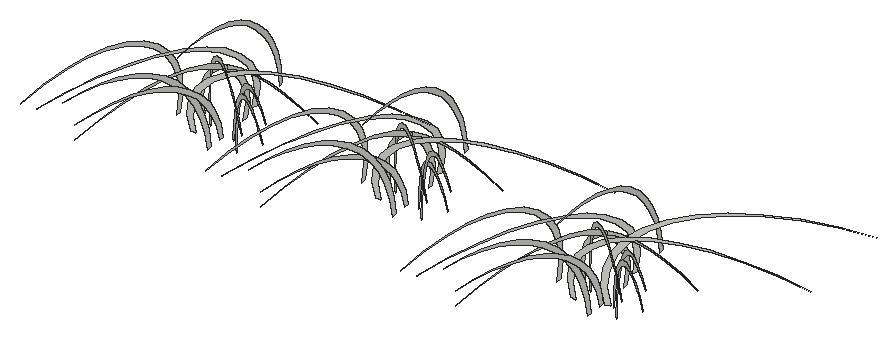
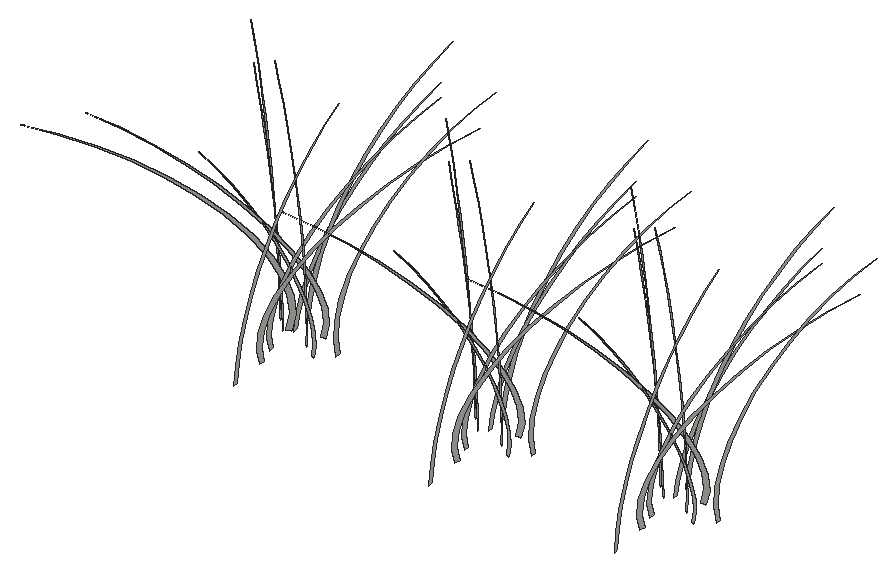
# SketchUp Ruby script. Lengths in inches.
U = 1.inch
M = Sketchup.active_model
def pt(a) = Geom::Point3d.new(a.map { |v| v * U })
def face(e, loops, mat)
  f = e.add_face(loops[0].map { |a| pt(a) })
  loops[1..].each { |l| e.add_face(l.map { |a| pt(a) }).erase! }
  f.material = f.back_material = mat if mat
  f
end
# faces: each face lists its corners as indices into pts; further lists are holes
def faces(e, pts, list, mat = nil) = list.each { |f| face(e, (f[0].is_a?(Array) ? f : [f]).map { |l| l.map { |i| pts[i] } }, mat) }
# xy, xz, yz: faces in a plane at the given z, y or x. An outline is a flat list of corners, or four numbers for a rectangle; further outlines are holes
def ring(l) = l.size == 4 ? [[l[0], l[1]], [l[2], l[1]], [l[2], l[3]], [l[0], l[3]]] : l.each_slice(2).to_a
def flat(e, list, mat, &to3) = list.each { |f| face(e, (f[0].is_a?(Array) ? f : [f]).map { |l| ring(l).map { |u, v| to3.(u, v) } }, mat) }
def xy(e, z, list, mat = nil) = flat(e, list, mat) { |x, y| [x, y, z] }
def xz(e, y, list, mat = nil) = flat(e, list, mat) { |x, z| [x, y, z] }
def yz(e, x, list, mat = nil) = flat(e, list, mat) { |y, z| [x, y, z] }
def lines(e, pts, list) = list.each { |a, b| e.add_line(pt(pts[a]), pt(pts[b])) }
# prism: a flat outline (further loops are holes) pulled along v
def prism(e, loops, v, mat = nil)
  f = face(e, loops, mat); d = Geom::Vector3d.new(v.map { |x| x * U })
  f.pushpull(f.normal.samedirection?(d) ? d.length : -d.length)
end
def box(e, o, s, mat = nil) = prism(e, [[o, [o[0] + s[0], o[1], o[2]], [o[0] + s[0], o[1] + s[1], o[2]], [o[0], o[1] + s[1], o[2]]]], [0, 0, s[2]], mat)
def at(x, y, z, deg = 0) = Geom::Transformation.translation(pt([x, y, z])) * Geom::Transformation.rotation(ORIGIN, Z_AXIS, deg.degrees)
def axes(o, x, y, z) = Geom::Transformation.new([*x, 0, *y, 0, *z, 0, *pt(o).to_a, 1])
def part(name) = M.definitions.add(name)
# library, detail: a bought-in or finely detailed component or shape, given as its bounding box
def library(name, o, s) = part(name).tap { |d| box(d.entities, o, s) }
def detail(e, o, s) = box(e.add_group.entities, o, s)
def put(e, d, t, mat = nil) = e.add_instance(d, t).tap { |i| i.material = mat if mat }
def group(e, t, mat = nil) = e.add_group.tap { |g| g.transformation = t; g.material = mat if mat }.entities
root = M.entities
g1 = group(root,at(472.64,259.22,0))
p = [[0.12,-0.92,0],[0.05,-0.41,0],[0,0,1.75],[0.02,-0.16,3.51],[0.11,-0.9,5.24],[0.27,-2.18,6.89],
  [0.5,-3.98,8.42],[0.79,-6.26,9.8],[1.13,-8.95,10.98],[1.51,-12,11.95],[1.93,-15.32,12.67],[2.37,-18.83,13.13],
  [2.83,-22.45,13.32],[3.28,-26.08,13.23],[2.84,-22.52,13.25],[2.39,-18.99,13],[1.96,-15.57,12.5],[1.56,-12.36,11.75],
  [1.19,-9.41,10.78],[0.86,-6.8,9.6],[0.58,-4.59,8.25],[0.36,-2.83,6.75],[0.2,-1.56,5.13],[0.1,-0.81,3.44],
  [0.07,-0.59,1.72]]
faces(g1,p,[[0,1,2,3,4,5,6,7,8,9,10,11,12,13,14,15,16,17,18,19,20,21,22,23,24]])
g2 = group(root,at(476.99,264.25,0))
p = [[-0.06,-0.99,0],[-0.03,-0.44,0],[0,0,1.49],[-0.01,-0.18,2.99],[-0.06,-0.97,4.45],[-0.14,-2.36,5.86],
  [-0.26,-4.3,7.16],[-0.4,-6.76,8.33],[-0.58,-9.67,9.33],[-0.77,-12.96,10.15],[-0.99,-16.54,10.77],[-1.22,-20.34,11.16],
  [-1.45,-24.24,11.32],[-1.68,-28.17,11.24],[-1.45,-24.32,11.26],[-1.23,-20.51,11.05],[-1.01,-16.82,10.625],[-0.8,-13.35,9.99],
  [-0.61,-10.16,9.16],[-0.4375,-7.35,8.16],[-0.3,-4.96,7.01],[-0.18,-3.06,5.73],[-0.1,-1.69,4.36],[-0.05,-0.87,2.93],
  [-0.04,-0.64,1.46]]
faces(g2,p,[[0,1,2,3,4,5,6,7,8,9,10,11,12,13,14,15,16,17,18,19,20,21,22,23,24]])
g3 = group(root,at(477.64,262,0))
p = [[0.125,-0.99,0],[0.06,-0.4375,0],[0,0,1.49],[0.02,-0.18,2.99],[0.12,-0.96,4.45],[0.3,-2.34,5.86],
  [0.54,-4.28,7.16],[0.85,-6.72,8.33],[1.21,-9.61,9.33],[1.62,-12.88,10.15],[2.07,-16.44,10.77],[2.55,-20.21,11.16],
  [3.03,-24.1,11.32],[3.53,-28,11.24],[3.04,-24.17,11.26],[2.57,-20.38,11.05],[2.11,-16.72,10.625],[1.67,-13.27,9.99],
  [1.27,-10.1,9.16],[0.92,-7.3,8.16],[0.62,-4.93,7.01],[0.38,-3.04,5.73],[0.21,-1.67,4.36],[0.11,-0.87,2.93],
  [0.08,-0.64,1.46]]
faces(g3,p,[[0,1,2,3,4,5,6,7,8,9,10,11,12,13,14,15,16,17,18,19,20,21,22,23,24]])
g4 = group(root,at(478.18,257.72,0))
p = [[2.6,-20.61,12.375],[2.99,-23.72,12.7],[2.61,-20.71,12.31],[2.24,-17.8,11.76],[1.89,-15.03,11.07],[1.56,-12.42,10.23],
  [1.26,-10.01,9.27],[0.99,-7.82,8.2],[0.74,-5.88,7.01],[0.53,-4.21,5.74],[0.36,-2.83,4.38],[0.22,-1.74,2.96],
  [0.125,-0.98,1.5],[0.07,-0.54,0],[0,0,0],[0.05,-0.36,1.53],[0.14,-1.08,3.03],[0.27,-2.14,4.49],
  [0.45,-3.54,5.875],[0.66,-5.24,7.18],[0.91,-7.24,8.375],[1.2,-9.51,9.46],[1.51,-12.01,10.41],[1.85,-14.72,11.22],
  [2.22,-17.6,11.88]]
faces(g4,p,[[0,1,2,3,4,5,6,7,8,9,10,11,12,13,14,15,16,17,18,19,20,21,22,23,24]])
g5 = group(root,at(476.24,268.1875,0))
p = [[6.07,-19.87,14.56],[6.99,-22.87,14.94],[6.1,-19.96,14.48],[5.25,-17.16,13.83],[4.43,-14.49,13.02],[3.66,-11.97,12.04],
  [2.95,-9.65,10.91],[2.31,-7.54,9.64],[1.73,-5.67,8.25],[1.24,-4.06,6.75],[0.83,-2.72,5.15],[0.51,-1.68,3.49],
  [0.29,-0.94,1.76],[0.16,-0.52,0],[0,0,0],[0.11,-0.35,1.8],[0.32,-1.04,3.57],[0.63,-2.07,5.28],
  [1.04,-3.41,6.91],[1.55,-5.05,8.44],[2.13,-6.98,9.85],[2.8,-9.16,11.13],[3.54,-11.58,12.25],[4.34,-14.1875,13.2],
  [5.1875,-16.96,13.97]]
faces(g5,p,[[0,1,2,3,4,5,6,7,8,9,10,11,12,13,14,15,16,17,18,19,20,21,22,23,24]])
g6 = group(root,at(478.42,255.81,0))
p = [[2.6,-20.61,15.34],[2.99,-23.72,15.75],[2.61,-20.71,15.26],[2.24,-17.8,14.58],[1.89,-15.03,13.72],[1.56,-12.42,12.69],
  [1.26,-10.01,11.5],[0.99,-7.82,10.16],[0.74,-5.88,8.7],[0.53,-4.21,7.11],[0.36,-2.83,5.43],[0.22,-1.74,3.67],
  [0.125,-0.98,1.86],[0.07,-0.54,0],[0,0,0],[0.05,-0.36,1.9],[0.14,-1.08,3.76],[0.27,-2.14,5.57],
  [0.45,-3.54,7.28],[0.66,-5.24,8.9],[0.91,-7.24,10.39],[1.2,-9.51,11.73],[1.51,-12.01,12.91],[1.85,-14.72,13.91],
  [2.22,-17.6,14.73]]
faces(g6,p,[[0,1,2,3,4,5,6,7,8,9,10,11,12,13,14,15,16,17,18,19,20,21,22,23,24]])
g7 = group(root,at(473.73,260.27,0))
p = [[0.69,-0.31,0],[0.31,-0.14,0],[0,0,1.24],[0.125,-0.06,2.49],[0.68,-0.3,3.72],[1.65,-0.73,4.89],
  [3.01,-1.34,5.98],[4.73,-2.11,6.95],[6.76,-3.01,7.8],[9.06,-4.04,8.48],[11.5625,-5.15,8.99],[14.21,-6.33,9.32],
  [16.94,-7.55,9.46],[19.6875,-8.77,9.39],[17,-7.58,9.4],[14.33,-6.39,9.23],[11.76,-5.24,8.875],[9.33,-4.16,8.35],
  [7.1,-3.17,7.65],[5.14,-2.29,6.82],[3.47,-1.55,5.86],[2.14,-0.95,4.79],[1.18,-0.52,3.64],[0.61,-0.27,2.45],
  [0.45,-0.2,1.22]]
faces(g7,p,[[0,1,2,3,4,5,6,7,8,9,10,11,12,13,14,15,16,17,18,19,20,21,22,23,24]])
g8 = group(root,at(475.44,259.31,0))
p = [[0.65,-0.66,0],[0.29,-0.29,0],[0,0,1.75],[0.12,-0.12,3.51],[0.64,-0.64,5.24],[1.55,-1.5625,6.89],
  [2.82,-2.86,8.42],[4.4375,-4.49,9.8],[6.35,-6.42,10.98],[8.5,-8.6,11.95],[10.85,-10.98,12.67],[13.34,-13.49,13.13],
  [15.91,-16.09,13.32],[18.48,-18.69,13.23],[15.96,-16.14,13.25],[13.45,-13.61,13],[11.04,-11.16,12.5],[8.76,-8.86,11.75],
  [6.67,-6.74,10.78],[4.82,-4.875,9.6],[3.25,-3.29,8.25],[2.01,-2.03,6.75],[1.11,-1.12,5.13],[0.57,-0.58,3.44],
  [0.42,-0.42,1.72]]
faces(g8,p,[[0,1,2,3,4,5,6,7,8,9,10,11,12,13,14,15,16,17,18,19,20,21,22,23,24]])
g9 = group(root,at(478.95,258.18,0))
p = [[14.61,-14.77,12.375],[16.8125,-17,12.7],[14.68,-14.84,12.31],[12.62,-12.76,11.76],[10.65,-10.77,11.07],[8.8,-8.9,10.23],
  [7.09,-7.17,9.27],[5.54,-5.61,8.2],[4.17,-4.22,7.01],[2.98,-3.02,5.74],[2,-2.02,4.38],[1.24,-1.25,2.96],
  [0.69,-0.7,1.5],[0.38,-0.38,0],[0,0,0],[0.26,-0.26,1.53],[0.77,-0.77,3.03],[1.52,-1.54,4.49],
  [2.51,-2.53,5.875],[3.72,-3.76,7.18],[5.13,-5.19,8.375],[6.74,-6.8125,9.46],[8.51,-8.61,10.41],[10.43,-10.55,11.22],
  [12.47,-12.61,11.88]]
faces(g9,p,[[0,1,2,3,4,5,6,7,8,9,10,11,12,13,14,15,16,17,18,19,20,21,22,23,24]])
g10 = group(root,at(480.3125,256.81,0))
p = [[14.61,-14.77,15.34],[16.8125,-17,15.75],[14.68,-14.84,15.26],[12.62,-12.76,14.58],[10.65,-10.77,13.72],[8.8,-8.9,12.69],
  [7.09,-7.17,11.5],[5.54,-5.61,10.16],[4.17,-4.22,8.7],[2.98,-3.02,7.11],[2,-2.02,5.43],[1.24,-1.25,3.67],
  [0.69,-0.7,1.86],[0.38,-0.38,0],[0,0,0],[0.26,-0.26,1.9],[0.77,-0.77,3.76],[1.52,-1.54,5.57],
  [2.51,-2.53,7.28],[3.72,-3.76,8.9],[5.13,-5.19,10.39],[6.74,-6.8125,11.73],[8.51,-8.61,12.91],[10.43,-10.55,13.91],
  [12.47,-12.61,14.73]]
faces(g10,p,[[0,1,2,3,4,5,6,7,8,9,10,11,12,13,14,15,16,17,18,19,20,21,22,23,24]])
g11 = group(root,at(474.92,256.97,0))
p = [[0.99,-0.08,0],[0.44,-0.04,0],[0,0,1.49],[0.18,-0.01,2.99],[0.97,-0.08,4.45],[2.35,-0.19,5.86],
  [4.3,-0.35,7.16],[6.75,-0.55,8.33],[9.66,-0.78,9.33],[12.9375,-1.05,10.15],[16.52,-1.34,10.77],[20.31,-1.64,11.16],
  [24.21,-1.96,11.32],[28.13,-2.27,11.24],[24.28,-1.96,11.26],[20.48,-1.66,11.05],[16.8,-1.36,10.625],[13.33,-1.08,9.99],
  [10.15,-0.82,9.16],[7.34,-0.59,8.16],[4.95,-0.4,7.01],[3.05,-0.25,5.73],[1.68,-0.14,4.36],[0.87,-0.07,2.93],
  [0.64,-0.05,1.46]]
faces(g11,p,[[0,1,2,3,4,5,6,7,8,9,10,11,12,13,14,15,16,17,18,19,20,21,22,23,24]])
g12 = group(root,at(492.11,259.95,0))
p = [[0.12,-0.92,0],[0.05,-0.41,0],[0,0,1.75],[0.02,-0.16,3.51],[0.11,-0.9,5.24],[0.27,-2.18,6.89],
  [0.5,-3.98,8.42],[0.79,-6.26,9.8],[1.13,-8.95,10.98],[1.51,-12,11.95],[1.93,-15.32,12.67],[2.37,-18.83,13.13],
  [2.83,-22.45,13.32],[3.28,-26.08,13.23],[2.84,-22.52,13.25],[2.39,-18.99,13],[1.96,-15.57,12.5],[1.56,-12.36,11.75],
  [1.19,-9.41,10.78],[0.86,-6.8,9.6],[0.58,-4.59,8.25],[0.36,-2.83,6.75],[0.2,-1.56,5.13],[0.1,-0.81,3.44],
  [0.07,-0.59,1.72]]
faces(g12,p,[[0,1,2,3,4,5,6,7,8,9,10,11,12,13,14,15,16,17,18,19,20,21,22,23,24]])
g13 = group(root,at(496.46,264.98,0))
p = [[-0.06,-0.99,0],[-0.03,-0.44,0],[0,0,1.49],[-0.01,-0.18,2.99],[-0.06,-0.97,4.45],[-0.14,-2.36,5.86],
  [-0.26,-4.3,7.16],[-0.4,-6.76,8.33],[-0.58,-9.67,9.33],[-0.77,-12.96,10.15],[-0.99,-16.54,10.77],[-1.22,-20.34,11.16],
  [-1.45,-24.24,11.32],[-1.68,-28.17,11.24],[-1.45,-24.32,11.26],[-1.23,-20.51,11.05],[-1.01,-16.82,10.625],[-0.8,-13.35,9.99],
  [-0.61,-10.16,9.16],[-0.4375,-7.35,8.16],[-0.3,-4.96,7.01],[-0.18,-3.06,5.73],[-0.1,-1.69,4.36],[-0.05,-0.87,2.93],
  [-0.04,-0.64,1.46]]
faces(g13,p,[[0,1,2,3,4,5,6,7,8,9,10,11,12,13,14,15,16,17,18,19,20,21,22,23,24]])
g14 = group(root,at(497.12,262.73,0))
p = [[0.125,-0.99,0],[0.06,-0.4375,0],[0,0,1.49],[0.02,-0.18,2.99],[0.12,-0.96,4.45],[0.3,-2.34,5.86],
  [0.54,-4.28,7.16],[0.85,-6.72,8.33],[1.21,-9.61,9.33],[1.62,-12.88,10.15],[2.07,-16.44,10.77],[2.55,-20.21,11.16],
  [3.03,-24.1,11.32],[3.53,-28,11.24],[3.04,-24.17,11.26],[2.57,-20.38,11.05],[2.11,-16.72,10.625],[1.67,-13.27,9.99],
  [1.27,-10.1,9.16],[0.92,-7.3,8.16],[0.62,-4.93,7.01],[0.38,-3.04,5.73],[0.21,-1.67,4.36],[0.11,-0.87,2.93],
  [0.08,-0.64,1.46]]
faces(g14,p,[[0,1,2,3,4,5,6,7,8,9,10,11,12,13,14,15,16,17,18,19,20,21,22,23,24]])
g15 = group(root,at(497.65,258.46,0))
p = [[2.6,-20.61,12.375],[2.99,-23.72,12.7],[2.61,-20.71,12.31],[2.24,-17.8,11.76],[1.89,-15.03,11.07],[1.56,-12.42,10.23],
  [1.26,-10.01,9.27],[0.99,-7.82,8.2],[0.74,-5.88,7.01],[0.53,-4.21,5.74],[0.36,-2.83,4.38],[0.22,-1.74,2.96],
  [0.125,-0.98,1.5],[0.07,-0.54,0],[0,0,0],[0.05,-0.36,1.53],[0.14,-1.08,3.03],[0.27,-2.14,4.49],
  [0.45,-3.54,5.875],[0.66,-5.24,7.18],[0.91,-7.24,8.375],[1.2,-9.51,9.46],[1.51,-12.01,10.41],[1.85,-14.72,11.22],
  [2.22,-17.6,11.88]]
faces(g15,p,[[0,1,2,3,4,5,6,7,8,9,10,11,12,13,14,15,16,17,18,19,20,21,22,23,24]])
g16 = group(root,at(495.72,268.92,0))
p = [[6.07,-19.87,14.56],[6.99,-22.87,14.94],[6.1,-19.96,14.48],[5.25,-17.16,13.83],[4.43,-14.49,13.02],[3.66,-11.97,12.04],
  [2.95,-9.65,10.91],[2.31,-7.54,9.64],[1.73,-5.67,8.25],[1.24,-4.06,6.75],[0.83,-2.72,5.15],[0.51,-1.68,3.49],
  [0.29,-0.94,1.76],[0.16,-0.52,0],[0,0,0],[0.11,-0.35,1.8],[0.32,-1.04,3.57],[0.63,-2.07,5.28],
  [1.04,-3.41,6.91],[1.55,-5.05,8.44],[2.13,-6.98,9.85],[2.8,-9.16,11.13],[3.54,-11.58,12.25],[4.34,-14.1875,13.2],
  [5.1875,-16.96,13.97]]
faces(g16,p,[[0,1,2,3,4,5,6,7,8,9,10,11,12,13,14,15,16,17,18,19,20,21,22,23,24]])
g17 = group(root,at(497.9,256.54,0))
p = [[2.6,-20.61,15.34],[2.99,-23.72,15.75],[2.61,-20.71,15.26],[2.24,-17.8,14.58],[1.89,-15.03,13.72],[1.56,-12.42,12.69],
  [1.26,-10.01,11.5],[0.99,-7.82,10.16],[0.74,-5.88,8.7],[0.53,-4.21,7.11],[0.36,-2.83,5.43],[0.22,-1.74,3.67],
  [0.125,-0.98,1.86],[0.07,-0.54,0],[0,0,0],[0.05,-0.36,1.9],[0.14,-1.08,3.76],[0.27,-2.14,5.57],
  [0.45,-3.54,7.28],[0.66,-5.24,8.9],[0.91,-7.24,10.39],[1.2,-9.51,11.73],[1.51,-12.01,12.91],[1.85,-14.72,13.91],
  [2.22,-17.6,14.73]]
faces(g17,p,[[0,1,2,3,4,5,6,7,8,9,10,11,12,13,14,15,16,17,18,19,20,21,22,23,24]])
g18 = group(root,at(493.2,261,0))
p = [[0.69,-0.31,0],[0.31,-0.14,0],[0,0,1.24],[0.125,-0.06,2.49],[0.68,-0.3,3.72],[1.65,-0.73,4.89],
  [3.01,-1.34,5.98],[4.73,-2.11,6.95],[6.76,-3.01,7.8],[9.06,-4.04,8.48],[11.5625,-5.15,8.99],[14.21,-6.33,9.32],
  [16.94,-7.55,9.46],[19.6875,-8.77,9.39],[17,-7.58,9.4],[14.33,-6.39,9.23],[11.76,-5.24,8.875],[9.33,-4.16,8.35],
  [7.1,-3.17,7.65],[5.14,-2.29,6.82],[3.47,-1.55,5.86],[2.14,-0.95,4.79],[1.18,-0.52,3.64],[0.61,-0.27,2.45],
  [0.45,-0.2,1.22]]
faces(g18,p,[[0,1,2,3,4,5,6,7,8,9,10,11,12,13,14,15,16,17,18,19,20,21,22,23,24]])
g19 = group(root,at(494.91,260.05,0))
p = [[0.65,-0.66,0],[0.29,-0.29,0],[0,0,1.75],[0.12,-0.12,3.51],[0.64,-0.64,5.24],[1.55,-1.5625,6.89],
  [2.82,-2.86,8.42],[4.4375,-4.49,9.8],[6.35,-6.42,10.98],[8.5,-8.6,11.95],[10.85,-10.98,12.67],[13.34,-13.49,13.13],
  [15.91,-16.09,13.32],[18.48,-18.69,13.23],[15.96,-16.14,13.25],[13.45,-13.61,13],[11.04,-11.16,12.5],[8.76,-8.86,11.75],
  [6.67,-6.74,10.78],[4.82,-4.875,9.6],[3.25,-3.29,8.25],[2.01,-2.03,6.75],[1.11,-1.12,5.13],[0.57,-0.58,3.44],
  [0.42,-0.42,1.72]]
faces(g19,p,[[0,1,2,3,4,5,6,7,8,9,10,11,12,13,14,15,16,17,18,19,20,21,22,23,24]])
g20 = group(root,at(498.43,258.92,0))
p = [[14.61,-14.77,12.375],[16.8125,-17,12.7],[14.68,-14.84,12.31],[12.62,-12.76,11.76],[10.65,-10.77,11.07],[8.8,-8.9,10.23],
  [7.09,-7.17,9.27],[5.54,-5.61,8.2],[4.17,-4.22,7.01],[2.98,-3.02,5.74],[2,-2.02,4.38],[1.24,-1.25,2.96],
  [0.69,-0.7,1.5],[0.38,-0.38,0],[0,0,0],[0.26,-0.26,1.53],[0.77,-0.77,3.03],[1.52,-1.54,4.49],
  [2.51,-2.53,5.875],[3.72,-3.76,7.18],[5.13,-5.19,8.375],[6.74,-6.8125,9.46],[8.51,-8.61,10.41],[10.43,-10.55,11.22],
  [12.47,-12.61,11.88]]
faces(g20,p,[[0,1,2,3,4,5,6,7,8,9,10,11,12,13,14,15,16,17,18,19,20,21,22,23,24]])
g21 = group(root,at(499.79,257.54,0))
p = [[14.61,-14.77,15.34],[16.8125,-17,15.75],[14.68,-14.84,15.26],[12.62,-12.76,14.58],[10.65,-10.77,13.72],[8.8,-8.9,12.69],
  [7.09,-7.17,11.5],[5.54,-5.61,10.16],[4.17,-4.22,8.7],[2.98,-3.02,7.11],[2,-2.02,5.43],[1.24,-1.25,3.67],
  [0.69,-0.7,1.86],[0.38,-0.38,0],[0,0,0],[0.26,-0.26,1.9],[0.77,-0.77,3.76],[1.52,-1.54,5.57],
  [2.51,-2.53,7.28],[3.72,-3.76,8.9],[5.13,-5.19,10.39],[6.74,-6.8125,11.73],[8.51,-8.61,12.91],[10.43,-10.55,13.91],
  [12.47,-12.61,14.73]]
faces(g21,p,[[0,1,2,3,4,5,6,7,8,9,10,11,12,13,14,15,16,17,18,19,20,21,22,23,24]])
g22 = group(root,at(494.39,257.7,0))
p = [[0.99,-0.08,0],[0.44,-0.04,0],[0,0,1.49],[0.18,-0.01,2.99],[0.97,-0.08,4.45],[2.35,-0.19,5.86],
  [4.3,-0.35,7.16],[6.75,-0.55,8.33],[9.66,-0.78,9.33],[12.9375,-1.05,10.15],[16.52,-1.34,10.77],[20.31,-1.64,11.16],
  [24.21,-1.96,11.32],[28.13,-2.27,11.24],[24.28,-1.96,11.26],[20.48,-1.66,11.05],[16.8,-1.36,10.625],[13.33,-1.08,9.99],
  [10.15,-0.82,9.16],[7.34,-0.59,8.16],[4.95,-0.4,7.01],[3.05,-0.25,5.73],[1.68,-0.14,4.36],[0.87,-0.07,2.93],
  [0.64,-0.05,1.46]]
faces(g22,p,[[0,1,2,3,4,5,6,7,8,9,10,11,12,13,14,15,16,17,18,19,20,21,22,23,24]])
g23 = group(root,at(515.69,256.89,0))
p = [[0.12,-0.92,0],[0.05,-0.41,0],[0,0,1.75],[0.02,-0.16,3.51],[0.11,-0.9,5.24],[0.27,-2.18,6.89],
  [0.5,-3.98,8.42],[0.79,-6.26,9.8],[1.13,-8.95,10.98],[1.51,-12,11.95],[1.93,-15.32,12.67],[2.37,-18.83,13.13],
  [2.83,-22.45,13.32],[3.28,-26.08,13.23],[2.84,-22.52,13.25],[2.39,-18.99,13],[1.96,-15.57,12.5],[1.56,-12.36,11.75],
  [1.19,-9.41,10.78],[0.86,-6.8,9.6],[0.58,-4.59,8.25],[0.36,-2.83,6.75],[0.2,-1.56,5.13],[0.1,-0.81,3.44],
  [0.07,-0.59,1.72]]
faces(g23,p,[[0,1,2,3,4,5,6,7,8,9,10,11,12,13,14,15,16,17,18,19,20,21,22,23,24]])
g24 = group(root,at(520.03,261.92,0))
p = [[-0.06,-0.99,0],[-0.03,-0.44,0],[0,0,1.49],[-0.01,-0.18,2.99],[-0.06,-0.97,4.45],[-0.14,-2.36,5.86],
  [-0.26,-4.3,7.16],[-0.4,-6.76,8.33],[-0.58,-9.67,9.33],[-0.77,-12.96,10.15],[-0.99,-16.54,10.77],[-1.22,-20.34,11.16],
  [-1.45,-24.24,11.32],[-1.68,-28.17,11.24],[-1.45,-24.32,11.26],[-1.23,-20.51,11.05],[-1.01,-16.82,10.625],[-0.8,-13.35,9.99],
  [-0.61,-10.16,9.16],[-0.4375,-7.35,8.16],[-0.3,-4.96,7.01],[-0.18,-3.06,5.73],[-0.1,-1.69,4.36],[-0.05,-0.87,2.93],
  [-0.04,-0.64,1.46]]
faces(g24,p,[[0,1,2,3,4,5,6,7,8,9,10,11,12,13,14,15,16,17,18,19,20,21,22,23,24]])
g25 = group(root,at(520.69,259.67,0))
p = [[0.125,-0.99,0],[0.06,-0.4375,0],[0,0,1.49],[0.02,-0.18,2.99],[0.12,-0.96,4.45],[0.3,-2.34,5.86],
  [0.54,-4.28,7.16],[0.85,-6.72,8.33],[1.21,-9.61,9.33],[1.62,-12.88,10.15],[2.07,-16.44,10.77],[2.55,-20.21,11.16],
  [3.03,-24.1,11.32],[3.53,-28,11.24],[3.04,-24.17,11.26],[2.57,-20.38,11.05],[2.11,-16.72,10.625],[1.67,-13.27,9.99],
  [1.27,-10.1,9.16],[0.92,-7.3,8.16],[0.62,-4.93,7.01],[0.38,-3.04,5.73],[0.21,-1.67,4.36],[0.11,-0.87,2.93],
  [0.08,-0.64,1.46]]
faces(g25,p,[[0,1,2,3,4,5,6,7,8,9,10,11,12,13,14,15,16,17,18,19,20,21,22,23,24]])
g26 = group(root,at(521.23,255.4,0))
p = [[2.6,-20.61,12.375],[2.99,-23.72,12.7],[2.61,-20.71,12.31],[2.24,-17.8,11.76],[1.89,-15.03,11.07],[1.56,-12.42,10.23],
  [1.26,-10.01,9.27],[0.99,-7.82,8.2],[0.74,-5.88,7.01],[0.53,-4.21,5.74],[0.36,-2.83,4.38],[0.22,-1.74,2.96],
  [0.125,-0.98,1.5],[0.07,-0.54,0],[0,0,0],[0.05,-0.36,1.53],[0.14,-1.08,3.03],[0.27,-2.14,4.49],
  [0.45,-3.54,5.875],[0.66,-5.24,7.18],[0.91,-7.24,8.375],[1.2,-9.51,9.46],[1.51,-12.01,10.41],[1.85,-14.72,11.22],
  [2.22,-17.6,11.88]]
faces(g26,p,[[0,1,2,3,4,5,6,7,8,9,10,11,12,13,14,15,16,17,18,19,20,21,22,23,24]])
g27 = group(root,at(519.29,265.86,0))
p = [[6.07,-19.87,14.56],[6.99,-22.87,14.94],[6.1,-19.96,14.48],[5.25,-17.16,13.83],[4.43,-14.49,13.02],[3.66,-11.97,12.04],
  [2.95,-9.65,10.91],[2.31,-7.54,9.64],[1.73,-5.67,8.25],[1.24,-4.06,6.75],[0.83,-2.72,5.15],[0.51,-1.68,3.49],
  [0.29,-0.94,1.76],[0.16,-0.52,0],[0,0,0],[0.11,-0.35,1.8],[0.32,-1.04,3.57],[0.63,-2.07,5.28],
  [1.04,-3.41,6.91],[1.55,-5.05,8.44],[2.13,-6.98,9.85],[2.8,-9.16,11.13],[3.54,-11.58,12.25],[4.34,-14.1875,13.2],
  [5.1875,-16.96,13.97]]
faces(g27,p,[[0,1,2,3,4,5,6,7,8,9,10,11,12,13,14,15,16,17,18,19,20,21,22,23,24]])
g28 = group(root,at(521.47,253.48,0))
p = [[2.6,-20.61,15.34],[2.99,-23.72,15.75],[2.61,-20.71,15.26],[2.24,-17.8,14.58],[1.89,-15.03,13.72],[1.56,-12.42,12.69],
  [1.26,-10.01,11.5],[0.99,-7.82,10.16],[0.74,-5.88,8.7],[0.53,-4.21,7.11],[0.36,-2.83,5.43],[0.22,-1.74,3.67],
  [0.125,-0.98,1.86],[0.07,-0.54,0],[0,0,0],[0.05,-0.36,1.9],[0.14,-1.08,3.76],[0.27,-2.14,5.57],
  [0.45,-3.54,7.28],[0.66,-5.24,8.9],[0.91,-7.24,10.39],[1.2,-9.51,11.73],[1.51,-12.01,12.91],[1.85,-14.72,13.91],
  [2.22,-17.6,14.73]]
faces(g28,p,[[0,1,2,3,4,5,6,7,8,9,10,11,12,13,14,15,16,17,18,19,20,21,22,23,24]])
g29 = group(root,at(516.78,257.94,0))
p = [[0.69,-0.31,0],[0.31,-0.14,0],[0,0,1.24],[0.125,-0.06,2.49],[0.68,-0.3,3.72],[1.65,-0.73,4.89],
  [3.01,-1.34,5.98],[4.73,-2.11,6.95],[6.76,-3.01,7.8],[9.06,-4.04,8.48],[11.5625,-5.15,8.99],[14.21,-6.33,9.32],
  [16.94,-7.55,9.46],[19.6875,-8.77,9.39],[17,-7.58,9.4],[14.33,-6.39,9.23],[11.76,-5.24,8.875],[9.33,-4.16,8.35],
  [7.1,-3.17,7.65],[5.14,-2.29,6.82],[3.47,-1.55,5.86],[2.14,-0.95,4.79],[1.18,-0.52,3.64],[0.61,-0.27,2.45],
  [0.45,-0.2,1.22]]
faces(g29,p,[[0,1,2,3,4,5,6,7,8,9,10,11,12,13,14,15,16,17,18,19,20,21,22,23,24]])
g30 = group(root,at(518.48,256.98,0))
p = [[0.65,-0.66,0],[0.29,-0.29,0],[0,0,1.75],[0.12,-0.12,3.51],[0.64,-0.64,5.24],[1.55,-1.5625,6.89],
  [2.82,-2.86,8.42],[4.4375,-4.49,9.8],[6.35,-6.42,10.98],[8.5,-8.6,11.95],[10.85,-10.98,12.67],[13.34,-13.49,13.13],
  [15.91,-16.09,13.32],[18.48,-18.69,13.23],[15.96,-16.14,13.25],[13.45,-13.61,13],[11.04,-11.16,12.5],[8.76,-8.86,11.75],
  [6.67,-6.74,10.78],[4.82,-4.875,9.6],[3.25,-3.29,8.25],[2.01,-2.03,6.75],[1.11,-1.12,5.13],[0.57,-0.58,3.44],
  [0.42,-0.42,1.72]]
faces(g30,p,[[0,1,2,3,4,5,6,7,8,9,10,11,12,13,14,15,16,17,18,19,20,21,22,23,24]])
g31 = group(root,at(522,255.85,0))
p = [[14.61,-14.77,12.375],[16.8125,-17,12.7],[14.68,-14.84,12.31],[12.62,-12.76,11.76],[10.65,-10.77,11.07],[8.8,-8.9,10.23],
  [7.09,-7.17,9.27],[5.54,-5.61,8.2],[4.17,-4.22,7.01],[2.98,-3.02,5.74],[2,-2.02,4.38],[1.24,-1.25,2.96],
  [0.69,-0.7,1.5],[0.38,-0.38,0],[0,0,0],[0.26,-0.26,1.53],[0.77,-0.77,3.03],[1.52,-1.54,4.49],
  [2.51,-2.53,5.875],[3.72,-3.76,7.18],[5.13,-5.19,8.375],[6.74,-6.8125,9.46],[8.51,-8.61,10.41],[10.43,-10.55,11.22],
  [12.47,-12.61,11.88]]
faces(g31,p,[[0,1,2,3,4,5,6,7,8,9,10,11,12,13,14,15,16,17,18,19,20,21,22,23,24]])
g32 = group(root,at(523.36,254.48,0))
p = [[14.61,-14.77,15.34],[16.8125,-17,15.75],[14.68,-14.84,15.26],[12.62,-12.76,14.58],[10.65,-10.77,13.72],[8.8,-8.9,12.69],
  [7.09,-7.17,11.5],[5.54,-5.61,10.16],[4.17,-4.22,8.7],[2.98,-3.02,7.11],[2,-2.02,5.43],[1.24,-1.25,3.67],
  [0.69,-0.7,1.86],[0.38,-0.38,0],[0,0,0],[0.26,-0.26,1.9],[0.77,-0.77,3.76],[1.52,-1.54,5.57],
  [2.51,-2.53,7.28],[3.72,-3.76,8.9],[5.13,-5.19,10.39],[6.74,-6.8125,11.73],[8.51,-8.61,12.91],[10.43,-10.55,13.91],
  [12.47,-12.61,14.73]]
faces(g32,p,[[0,1,2,3,4,5,6,7,8,9,10,11,12,13,14,15,16,17,18,19,20,21,22,23,24]])
g33 = group(root,at(517.97,254.64,0))
p = [[0.99,-0.08,0],[0.44,-0.04,0],[0,0,1.49],[0.18,-0.01,2.99],[0.97,-0.08,4.45],[2.35,-0.19,5.86],
  [4.3,-0.35,7.16],[6.75,-0.55,8.33],[9.66,-0.78,9.33],[12.9375,-1.05,10.15],[16.52,-1.34,10.77],[20.31,-1.64,11.16],
  [24.21,-1.96,11.32],[28.13,-2.27,11.24],[24.28,-1.96,11.26],[20.48,-1.66,11.05],[16.8,-1.36,10.625],[13.33,-1.08,9.99],
  [10.15,-0.82,9.16],[7.34,-0.59,8.16],[4.95,-0.4,7.01],[3.05,-0.25,5.73],[1.68,-0.14,4.36],[0.87,-0.07,2.93],
  [0.64,-0.05,1.46]]
faces(g33,p,[[0,1,2,3,4,5,6,7,8,9,10,11,12,13,14,15,16,17,18,19,20,21,22,23,24]])
g34 = group(root,at(521.05,255.34,0))
p = [[0.91,0.18,0],[0.4,0.08,0],[0,0,1.75],[0.16,0.03,3.51],[0.89,0.17,5.24],[2.16,0.42,6.89],
  [3.94,0.76,8.42],[6.19,1.2,9.8],[8.86,1.72,10.98],[11.87,2.3,11.95],[15.16,2.94,12.67],[18.63,3.61,13.13],
  [22.21,4.31,13.32],[25.81,5.01,13.23],[22.28,4.32,13.25],[18.79,3.64,13],[15.41,2.99,12.5],[12.23,2.37,11.75],
  [9.3125,1.81,10.78],[6.73,1.31,9.6],[4.54,0.88,8.25],[2.8,0.54,6.75],[1.54,0.3,5.13],[0.8,0.16,3.44],
  [0.59,0.11,1.72]]
faces(g34,p,[[0,1,2,3,4,5,6,7,8,9,10,11,12,13,14,15,16,17,18,19,20,21,22,23,24]])
